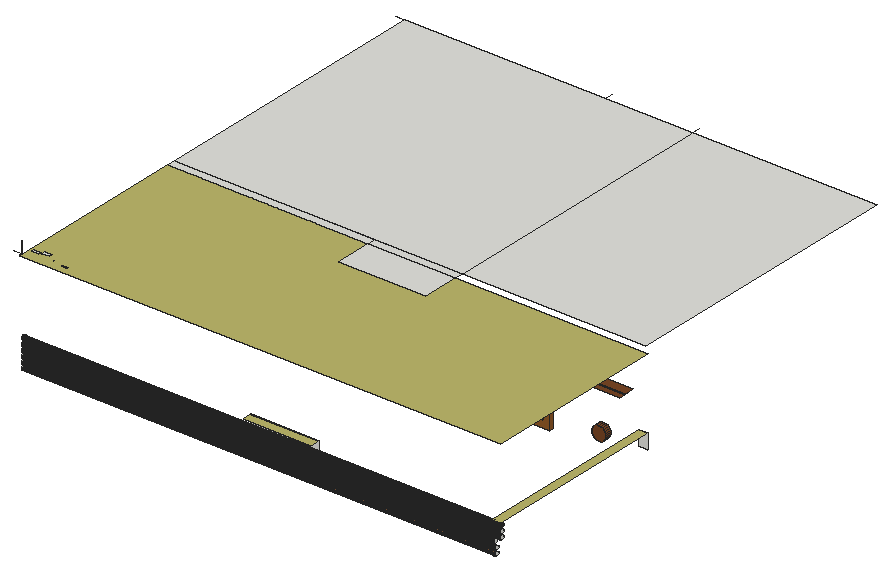
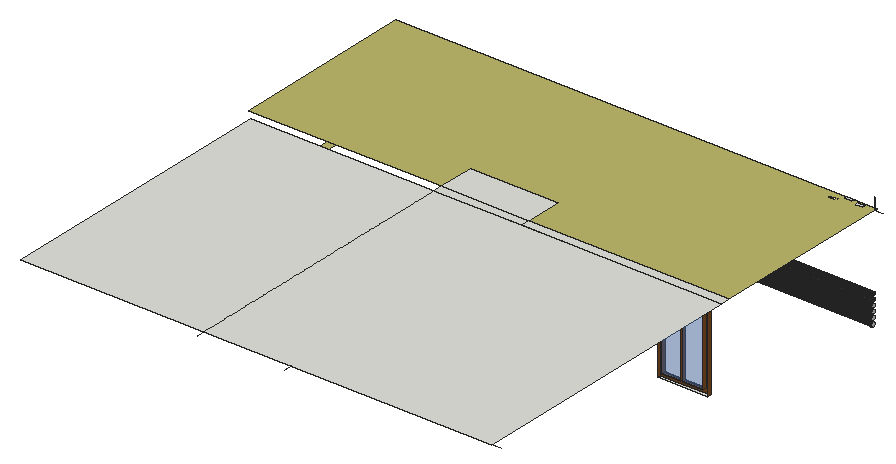
# SketchUp Ruby script. Lengths in inches.
U = 1.inch
M = Sketchup.active_model
def pt(a) = Geom::Point3d.new(a.map { |v| v * U })
def face(e, loops, mat)
  f = e.add_face(loops[0].map { |a| pt(a) })
  loops[1..].each { |l| e.add_face(l.map { |a| pt(a) }).erase! }
  f.material = f.back_material = mat if mat
  f
end
# faces: each face lists its corners as indices into pts; further lists are holes
def faces(e, pts, list, mat = nil) = list.each { |f| face(e, (f[0].is_a?(Array) ? f : [f]).map { |l| l.map { |i| pts[i] } }, mat) }
# xy, xz, yz: faces in a plane at the given z, y or x. An outline is a flat list of corners, or four numbers for a rectangle; further outlines are holes
def ring(l) = l.size == 4 ? [[l[0], l[1]], [l[2], l[1]], [l[2], l[3]], [l[0], l[3]]] : l.each_slice(2).to_a
def flat(e, list, mat, &to3) = list.each { |f| face(e, (f[0].is_a?(Array) ? f : [f]).map { |l| ring(l).map { |u, v| to3.(u, v) } }, mat) }
def xy(e, z, list, mat = nil) = flat(e, list, mat) { |x, y| [x, y, z] }
def xz(e, y, list, mat = nil) = flat(e, list, mat) { |x, z| [x, y, z] }
def yz(e, x, list, mat = nil) = flat(e, list, mat) { |y, z| [x, y, z] }
def lines(e, pts, list) = list.each { |a, b| e.add_line(pt(pts[a]), pt(pts[b])) }
# prism: a flat outline (further loops are holes) pulled along v
def prism(e, loops, v, mat = nil)
  f = face(e, loops, mat); d = Geom::Vector3d.new(v.map { |x| x * U })
  f.pushpull(f.normal.samedirection?(d) ? d.length : -d.length)
end
def box(e, o, s, mat = nil) = prism(e, [[o, [o[0] + s[0], o[1], o[2]], [o[0] + s[0], o[1] + s[1], o[2]], [o[0], o[1] + s[1], o[2]]]], [0, 0, s[2]], mat)
def at(x, y, z, deg = 0) = Geom::Transformation.translation(pt([x, y, z])) * Geom::Transformation.rotation(ORIGIN, Z_AXIS, deg.degrees)
def axes(o, x, y, z) = Geom::Transformation.new([*x, 0, *y, 0, *z, 0, *pt(o).to_a, 1])
def part(name) = M.definitions.add(name)
# library, detail: a bought-in or finely detailed component or shape, given as its bounding box
def library(name, o, s) = part(name).tap { |d| box(d.entities, o, s) }
def detail(e, o, s) = box(e.add_group.entities, o, s)
def put(e, d, t, mat = nil) = e.add_instance(d, t).tap { |i| i.material = mat if mat }
def group(e, t, mat = nil) = e.add_group.tap { |g| g.transformation = t; g.material = mat if mat }.entities
root = M.entities
M.materials.add("[0057_DarkKhaki]").color = [189, 183, 107]
M.materials.add("[Sandstone]").color = [118, 81, 52]
M.materials.add("[Translucent Glass Blue]").color = [100, 149, 237]
M.materials["[Translucent Glass Blue]"].alpha = 0.5
M.materials.add("[Wood Bamboo]").color = [177, 105, 43]
M.materials.add("[Wood Floor Parquet]").color = [145, 89, 39]
M.materials.add("[Wood Veneer 01]").color = [120, 70, 37]
xy(root,380.84,[[312.25,189.3,386.1875,192.3]],"[Wood Floor Parquet]")
xy(root,386.98,[[29.8125,189.3,79,192.3]])
xy(root,387.65,[[319.06,189.3,349.22,192.3],[353.36,189.3,379.38,192.3]],"[Wood Floor Parquet]")
xy(root,391.47,[[34.31,189.3,54.41,192.3],[56.03,189.3,74.5,192.3]],"[Wood Floor Parquet]")
xy(root,396.16,[[109.64,186.3,111.7,189.3]],"[Wood Bamboo]")
xy(root,401.1,[[96.64,186.3,109.64,189.3]],"[Wood Bamboo]")
xy(root,403.6,[[96.64,186.3,111.7,189.3]],"[Wood Bamboo]")
xy(root,410.4375,[[471.0625,12,480,192.3]],"[0057_DarkKhaki]")
xy(root,413.38,[[227.54,12,293.97,21]],"[0057_DarkKhaki]")
xy(root,429.52,[[123.78,186.3,171.53,189.3]],"[Wood Bamboo]")
xy(root,438.4,[[426.75,183.3,426.75,189.3,410.93,189.3,410.93,192.3,459.74,192.3,459.74,189.3,427.96,189.3,427.96,183.3]])
xy(root,438.4,[[410.93,183.3,426.75,189.3],[427.96,183.3,459.74,189.3]],"[Wood Veneer 01]")
xy(root,440.64,[[123.78,186.3,171.53,189.3]],"[Wood Bamboo]")
xy(root,444,[[116.27,186.3,119.49,186.3,119.49,189.3,176.74,189.3,176.74,192.3,92.74,192.3,92.74,189.3,116.27,189.3]],"[Wood Bamboo]")
xy(root,444,[[405.34,183.3,465.34,192.3]],"[Wood Veneer 01]")
xy(root,447.98,[[319.06,189.3,349.22,192.3],[353.36,189.3,379.38,192.3]],"[Wood Floor Parquet]")
xy(root,454.78,[[312.25,189.3,386.1875,192.3]],"[Wood Floor Parquet]")
xy(root,457.11,[[34.31,189.3,54.41,192.3],[56.03,189.3,74.5,192.3]],"[Wood Floor Parquet]")
xy(root,461.6,[[29.8125,189.3,79,192.3]],"[Wood Floor Parquet]")
xy(root,479.9375,[[34.65,18,41.83,21]])
xy(root,480,[[205.37,156.87,290.8125,192.3],[9,192.3,205.37,201.23],[205.37,192.3,290.8125,201.23],[9,201.23,290.8125,483],[290.8125,201.23,471,483]])
xy(root,480,[[[9,12,9,192.3,205.37,192.3,205.37,156.87,290.8125,156.87,290.8125,192.3,480,192.3,480,12],[42.9,18,50.08,21]]],"[0057_DarkKhaki]")
xy(root,483.12,[[15.02,18,22.21,21]])
xy(root,485,[[25.65,18,32.83,21]])
xz(root,21,[[227.54,389.38,293.97,413.38]])
xz(root,183.3,[[438.92,392.76,440.72,393,442.39,393.69,443.83,394.8,444.93,396.23,445.625,397.91,445.86,399.7,445.625,401.5,444.93,403.17,443.83,404.61,442.39,405.71,440.72,406.4,438.92,406.64,437.13,406.4,435.46,405.71,434.02,404.61,432.92,403.17,432.22,401.5,431.99,399.7,432.22,397.91,432.92,396.23,434.02,394.8,435.46,393.69,437.13,393]],"[Wood Veneer 01]")
xz(root,186.3,[[132.85,392.25,134.99,392.53,136.98,393.36,138.68,394.67,140,396.38,140.82,398.37,141.1,400.5,140.82,402.64,140,404.63,138.68,406.34,136.98,407.65,134.99,408.47,132.85,408.75,130.72,408.47,128.73,407.65,127.02,406.34,125.71,404.63,124.88,402.64,124.6,400.5,124.88,398.37,125.71,396.38,127.02,394.67,128.73,393.36,130.72,392.53],[109.64,396.16,111.7,396.16,111.7,403.6,96.64,403.6,96.64,401.1,109.64,401.1],[123.78,429.52,171.53,440.64]],"[Wood Bamboo]")
xz(root,189.3,[[109.64,396.16,109.64,401.1,96.64,401.1,96.64,403.6,111.7,403.6,111.7,396.16]])
xz(root,189.3,[[[119.49,422.86,176.74,444],[123.78,429.52,171.53,440.64]]],"[Wood Bamboo]")
xz(root,189.3,[[[312.25,380.84,386.1875,454.78],[319.06,387.65,349.22,447.98],[353.36,387.65,379.38,447.98]],[[29.8125,386.98,79,461.6],[34.31,391.47,54.41,457.11],[56.03,391.47,74.5,457.11]]],"[Wood Floor Parquet]")
xz(root,192.3,[[[312.25,380.84,386.1875,454.78],[319.06,387.65,349.22,447.98],[353.36,387.65,379.38,447.98]],[471.0625,396,480,410.4375]])
xz(root,192.3,[[319.06,387.65,349.22,447.98],[353.36,387.65,379.38,447.98],[34.31,391.47,54.41,457.11],[56.03,391.47,74.5,457.11]],"[Translucent Glass Blue]")
yz(root,9,[[15.36,378.27,14.91,378.33,14.49,378.5,14.125,378.78,13.85,379.14,13.67,379.5625,13.61,380.02,13.67,380.47,13.85,380.89,14.125,381.25,14.49,381.53,14.91,381.71,15.36,381.77,15.82,381.71,16.24,381.53,16.6,381.25,16.88,380.89,17.05,380.47,17.11,380.02,17.05,379.5625,16.88,379.14,16.6,378.78,16.24,378.5,15.82,378.33],[15.36,383.58,14.91,383.64,14.49,383.8125,14.125,384.09,13.85,384.45,13.67,384.875,13.61,385.33,13.67,385.78,13.85,386.2,14.125,386.57,14.49,386.84,14.91,387.02,15.36,387.08,15.82,387.02,16.24,386.84,16.6,386.57,16.88,386.2,17.05,385.78,17.11,385.33,17.05,384.875,16.88,384.45,16.6,384.09,16.24,383.8125,15.82,383.64],[15.36,388.89,14.91,388.95,14.49,389.125,14.125,389.4,13.85,389.77,13.67,390.1875,13.61,390.64,13.67,391.09,13.85,391.52,14.125,391.88,14.49,392.16,14.91,392.33,15.36,392.39,15.82,392.33,16.24,392.16,16.6,391.88,16.88,391.52,17.05,391.09,17.11,390.64,17.05,390.1875,16.88,389.77,16.6,389.4,16.24,389.125,15.82,388.95],[15.36,394.2,14.91,394.26,14.49,394.4375,14.125,394.72,13.85,395.08,13.67,395.5,13.61,395.95,13.67,396.41,13.85,396.83,14.125,397.19,14.49,397.47,14.91,397.64,15.36,397.7,15.82,397.64,16.24,397.47,16.6,397.19,16.88,396.83,17.05,396.41,17.11,395.95,17.05,395.5,16.88,395.08,16.6,394.72,16.24,394.4375,15.82,394.26]])
yz(root,29.8125,[[189.3,386.98,192.3,461.6]],"[Wood Floor Parquet]")
yz(root,34.31,[[189.3,391.47,192.3,457.11]],"[Wood Floor Parquet]")
yz(root,54.41,[[189.3,391.47,192.3,457.11]],"[Wood Floor Parquet]")
yz(root,56.03,[[189.3,391.47,192.3,457.11]],"[Wood Floor Parquet]")
yz(root,74.5,[[189.3,391.47,192.3,457.11]],"[Wood Floor Parquet]")
yz(root,79,[[189.3,386.98,192.3,461.6]],"[Wood Floor Parquet]")
yz(root,96.64,[[186.3,401.1,189.3,403.6]],"[Wood Bamboo]")
yz(root,109.64,[[186.3,396.16,189.3,401.1]],"[Wood Bamboo]")
yz(root,111.7,[[186.3,396.16,189.3,403.6]],"[Wood Bamboo]")
yz(root,123.78,[[186.3,429.52,189.3,440.64]],"[Wood Bamboo]")
yz(root,171.53,[[186.3,429.52,189.3,440.64]],"[Wood Bamboo]")
yz(root,312.25,[[189.3,380.84,192.3,454.78]],"[Wood Floor Parquet]")
yz(root,319.06,[[189.3,387.65,192.3,447.98]],"[Wood Floor Parquet]")
yz(root,349.22,[[189.3,387.65,192.3,447.98]],"[Wood Floor Parquet]")
yz(root,353.36,[[189.3,387.65,192.3,447.98]],"[Wood Floor Parquet]")
yz(root,379.38,[[189.3,387.65,192.3,447.98]],"[Wood Floor Parquet]")
yz(root,386.1875,[[189.3,380.84,192.3,454.78]],"[Wood Floor Parquet]")
yz(root,472.25,[[15.36,388.89,15.82,388.95,16.24,389.125,16.6,389.4,16.88,389.77,17.05,390.1875,17.11,390.64,17.05,391.09,16.88,391.52,16.6,391.88,16.24,392.16,15.82,392.33,15.36,392.39,14.91,392.33,14.49,392.16,14.125,391.88,13.85,391.52,13.67,391.09,13.61,390.64,13.67,390.1875,13.85,389.77,14.125,389.4,14.49,389.125,14.91,388.95]])
yz(root,473.625,[[15.36,378.27,15.82,378.33,16.24,378.5,16.6,378.78,16.88,379.14,17.05,379.5625,17.11,380.02,17.05,380.47,16.88,380.89,16.6,381.25,16.24,381.53,15.82,381.71,15.36,381.77,14.91,381.71,14.49,381.53,14.125,381.25,13.85,380.89,13.67,380.47,13.61,380.02,13.67,379.5625,13.85,379.14,14.125,378.78,14.49,378.5,14.91,378.33],[15.36,383.58,15.82,383.64,16.24,383.8125,16.6,384.09,16.88,384.45,17.05,384.875,17.11,385.33,17.05,385.78,16.88,386.2,16.6,386.57,16.24,386.84,15.82,387.02,15.36,387.08,14.91,387.02,14.49,386.84,14.125,386.57,13.85,386.2,13.67,385.78,13.61,385.33,13.67,384.875,13.85,384.45,14.125,384.09,14.49,383.8125,14.91,383.64]])
yz(root,478.4375,[[15.36,394.2,15.82,394.26,16.24,394.4375,16.6,394.72,16.88,395.08,17.05,395.5,17.11,395.95,17.05,396.41,16.88,396.83,16.6,397.19,16.24,397.47,15.82,397.64,15.36,397.7,14.91,397.64,14.49,397.47,14.125,397.19,13.85,396.83,13.67,396.41,13.61,395.95,13.67,395.5,13.85,395.08,14.125,394.72,14.49,394.4375,14.91,394.26],[15.36,399.52,15.82,399.58,16.24,399.75,16.6,400.03,16.88,400.39,17.05,400.8125,17.11,401.27,17.05,401.72,16.88,402.14,16.6,402.5,16.24,402.78,15.82,402.96,15.36,403.02,14.91,402.96,14.49,402.78,14.125,402.5,13.85,402.14,13.67,401.72,13.61,401.27,13.67,400.8125,13.85,400.39,14.125,400.03,14.49,399.75,14.91,399.58]])
p = [[9,14.49,378.5],[9,14.91,378.33],[473.625,14.91,378.33],[473.625,14.49,378.5],[9,15.36,378.27],[473.625,15.36,378.27],
  [9,15.82,378.33],[473.625,15.82,378.33],[9,16.24,378.5],[473.625,16.24,378.5],[9,14.125,378.78],[473.625,14.125,378.78],
  [9,16.6,378.78],[473.625,16.6,378.78],[9,13.85,379.14],[473.625,13.85,379.14],[9,16.88,379.14],[473.625,16.88,379.14],
  [9,13.67,379.5625],[473.625,13.67,379.5625],[9,17.05,379.5625],[473.625,17.05,379.5625],[9,13.61,380.02],[473.625,13.61,380.02],
  [9,17.11,380.02],[473.625,17.11,380.02],[9,13.67,380.47],[473.625,13.67,380.47],[9,17.05,380.47],[473.625,17.05,380.47],
  [9,13.85,380.89],[473.625,13.85,380.89],[9,16.88,380.89],[473.625,16.88,380.89],[9,14.125,381.25],[473.625,14.125,381.25],
  [9,16.6,381.25],[473.625,16.6,381.25],[9,14.49,381.53],[473.625,14.49,381.53],[9,16.24,381.53],[473.625,16.24,381.53],
  [9,14.91,381.71],[473.625,14.91,381.71],[9,15.82,381.71],[473.625,15.82,381.71],[9,15.36,381.77],[473.625,15.36,381.77],
  [9,14.49,383.8125],[9,14.91,383.64],[473.625,14.91,383.64],[473.625,14.49,383.8125],[9,15.36,383.58],[473.625,15.36,383.58],
  [9,15.82,383.64],[473.625,15.82,383.64],[9,16.24,383.8125],[473.625,16.24,383.8125],[9,14.125,384.09],[473.625,14.125,384.09],
  [9,16.6,384.09],[473.625,16.6,384.09],[9,13.85,384.45],[473.625,13.85,384.45],[9,16.88,384.45],[473.625,16.88,384.45],
  [9,13.67,384.875],[473.625,13.67,384.875],[9,17.05,384.875],[473.625,17.05,384.875],[9,13.61,385.33],[473.625,13.61,385.33],
  [9,17.11,385.33],[473.625,17.11,385.33],[9,13.67,385.78],[473.625,13.67,385.78],[9,17.05,385.78],[473.625,17.05,385.78],
  [9,13.85,386.2],[473.625,13.85,386.2],[9,16.88,386.2],[473.625,16.88,386.2],[9,14.125,386.57],[473.625,14.125,386.57],
  [9,16.6,386.57],[473.625,16.6,386.57],[9,14.49,386.84],[473.625,14.49,386.84],[9,16.24,386.84],[473.625,16.24,386.84],
  [9,14.91,387.02],[473.625,14.91,387.02],[9,15.82,387.02],[473.625,15.82,387.02],[9,15.36,387.08],[473.625,15.36,387.08],
  [9,14.91,388.95],[9,15.36,388.89],[472.25,15.36,388.89],[472.25,14.91,388.95],[9,15.82,388.95],[472.25,15.82,388.95],
  [9,14.49,389.125],[472.25,14.49,389.125],[9,16.24,389.125],[472.25,16.24,389.125],[9,14.125,389.4],[472.25,14.125,389.4],
  [9,16.6,389.4],[472.25,16.6,389.4],[9,13.85,389.77],[472.25,13.85,389.77],[9,16.88,389.77],[472.25,16.88,389.77],
  [9,13.67,390.1875],[472.25,13.67,390.1875],[9,17.05,390.1875],[472.25,17.05,390.1875],[9,13.61,390.64],[472.25,13.61,390.64],
  [9,17.11,390.64],[472.25,17.11,390.64],[9,13.67,391.09],[472.25,13.67,391.09],[9,17.05,391.09],[472.25,17.05,391.09],
  [9,13.85,391.52],[472.25,13.85,391.52],[9,16.88,391.52],[472.25,16.88,391.52],[9,14.125,391.88],[472.25,14.125,391.88],
  [9,16.6,391.88],[472.25,16.6,391.88],[9,14.49,392.16],[472.25,14.49,392.16],[9,16.24,392.16],[472.25,16.24,392.16],
  [9,14.91,392.33],[472.25,14.91,392.33],[9,15.82,392.33],[472.25,15.82,392.33],[9,15.36,392.39],[472.25,15.36,392.39],
  [130.72,189.3,392.53],[132.85,189.3,392.25],[132.85,186.3,392.25],[130.72,186.3,392.53],[134.99,189.3,392.53],[134.99,186.3,392.53],
  [128.73,189.3,393.36],[128.73,186.3,393.36],[136.98,189.3,393.36],[136.98,186.3,393.36],[437.13,189.3,393],[438.92,189.3,392.76],
  [438.92,183.3,392.76],[437.13,183.3,393],[440.72,189.3,393],[440.72,183.3,393],[435.46,189.3,393.69],[435.46,183.3,393.69],
  [442.39,189.3,393.69],[442.39,183.3,393.69],[127.02,189.3,394.67],[127.02,186.3,394.67],[138.68,189.3,394.67],[138.68,186.3,394.67],
  [434.02,189.3,394.8],[434.02,183.3,394.8],[443.83,189.3,394.8],[443.83,183.3,394.8],[9,14.91,394.26],[9,15.36,394.2],
  [478.4375,15.36,394.2],[478.4375,14.91,394.26],[9,15.82,394.26],[478.4375,15.82,394.26],[9,14.49,394.4375],[478.4375,14.49,394.4375],
  [9,16.24,394.4375],[478.4375,16.24,394.4375],[9,14.125,394.72],[478.4375,14.125,394.72],[9,16.6,394.72],[478.4375,16.6,394.72],
  [9,13.85,395.08],[478.4375,13.85,395.08],[9,16.88,395.08],[478.4375,16.88,395.08],[125.71,189.3,396.38],[125.71,186.3,396.38],
  [140,189.3,396.38],[140,186.3,396.38],[432.92,189.3,396.23],[432.92,183.3,396.23],[444.93,189.3,396.23],[444.93,183.3,396.23],
  [9,13.67,395.5],[478.4375,13.67,395.5],[9,17.05,395.5],[478.4375,17.05,395.5],[9,13.61,395.95],[478.4375,13.61,395.95],
  [9,17.11,395.95],[478.4375,17.11,395.95],[9,13.67,396.41],[478.4375,13.67,396.41],[9,17.05,396.41],[478.4375,17.05,396.41],
  [432.22,189.3,397.91],[432.22,183.3,397.91],[445.625,189.3,397.91],[445.625,183.3,397.91],[9,13.85,396.83],[478.4375,13.85,396.83],
  [9,16.88,396.83],[478.4375,16.88,396.83],[124.88,189.3,398.37],[124.88,186.3,398.37],[140.82,189.3,398.37],[140.82,186.3,398.37],
  [9,14.125,397.19],[478.4375,14.125,397.19],[9,16.6,397.19],[478.4375,16.6,397.19],[9,14.49,397.47],[478.4375,14.49,397.47],
  [9,16.24,397.47],[478.4375,16.24,397.47],[9,14.91,397.64],[478.4375,14.91,397.64],[9,15.82,397.64],[478.4375,15.82,397.64],
  [9,15.36,397.7],[478.4375,15.36,397.7],[431.99,189.3,399.7],[431.99,183.3,399.7],[445.86,189.3,399.7],[445.86,183.3,399.7],
  [124.6,189.3,400.5],[124.6,186.3,400.5],[141.1,189.3,400.5],[141.1,186.3,400.5],[9,14.91,399.58],[9,15.36,399.52],
  [478.4375,15.36,399.52],[478.4375,14.91,399.58],[9,15.82,399.58],[478.4375,15.82,399.58],[9,14.49,399.75],[478.4375,14.49,399.75],
  [9,16.24,399.75],[478.4375,16.24,399.75],[432.22,189.3,401.5],[432.22,183.3,401.5],[445.625,189.3,401.5],[445.625,183.3,401.5],
  [9,14.125,400.03],[478.4375,14.125,400.03],[9,16.6,400.03],[478.4375,16.6,400.03],[9,13.85,400.39],[478.4375,13.85,400.39],
  [9,16.88,400.39],[478.4375,16.88,400.39],[9,13.67,400.8125],[478.4375,13.67,400.8125],[9,17.05,400.8125],[478.4375,17.05,400.8125],
  [124.88,189.3,402.64],[124.88,186.3,402.64],[140.82,189.3,402.64],[140.82,186.3,402.64],[9,13.61,401.27],[478.4375,13.61,401.27],
  [9,17.11,401.27],[478.4375,17.11,401.27],[9,13.67,401.72],[478.4375,13.67,401.72],[9,17.05,401.72],[478.4375,17.05,401.72],
  [432.92,189.3,403.17],[432.92,183.3,403.17],[444.93,189.3,403.17],[444.93,183.3,403.17],[9,13.85,402.14],[478.4375,13.85,402.14],
  [9,16.88,402.14],[478.4375,16.88,402.14],[9,14.125,402.5],[478.4375,14.125,402.5],[9,16.6,402.5],[478.4375,16.6,402.5],
  [9,14.49,402.78],[478.4375,14.49,402.78],[9,16.24,402.78],[478.4375,16.24,402.78],[125.71,189.3,404.63],[125.71,186.3,404.63],
  [140,189.3,404.63],[140,186.3,404.63],[9,14.91,402.96],[478.4375,14.91,402.96],[9,15.82,402.96],[478.4375,15.82,402.96],
  [9,15.36,403.02],[478.4375,15.36,403.02],[434.02,189.3,404.61],[434.02,183.3,404.61],[443.83,189.3,404.61],[443.83,183.3,404.61],
  [435.46,189.3,405.71],[435.46,183.3,405.71],[442.39,189.3,405.71],[442.39,183.3,405.71],[127.02,189.3,406.34],[127.02,186.3,406.34],
  [138.68,189.3,406.34],[138.68,186.3,406.34],[9,14.49,405.1875],[9,14.91,405.01],[478.4375,14.91,405.01],[478.4375,14.49,405.1875],
  [9,15.36,404.95],[478.4375,15.36,404.95],[9,15.82,405.01],[478.4375,15.82,405.01],[9,16.24,405.1875],[478.4375,16.24,405.1875],
  [9,14.125,405.47],[478.4375,14.125,405.47],[9,16.6,405.47],[478.4375,16.6,405.47],[9,13.85,405.83],[478.4375,13.85,405.83],
  [9,16.88,405.83],[478.4375,16.88,405.83],[437.13,189.3,406.4],[437.13,183.3,406.4],[440.72,189.3,406.4],[440.72,183.3,406.4],
  [9,13.67,406.25],[478.4375,13.67,406.25],[9,17.05,406.25],[478.4375,17.05,406.25],[9,13.61,406.7],[478.4375,13.61,406.7],
  [9,17.11,406.7],[478.4375,17.11,406.7],[128.73,189.3,407.65],[128.73,186.3,407.65],[136.98,189.3,407.65],[136.98,186.3,407.65],
  [438.92,189.3,406.64],[438.92,183.3,406.64],[9,13.67,407.16],[478.4375,13.67,407.16],[9,17.05,407.16],[478.4375,17.05,407.16],
  [9,13.85,407.58],[478.4375,13.85,407.58],[9,16.88,407.58],[478.4375,16.88,407.58],[9,14.125,407.94],[478.4375,14.125,407.94],
  [9,16.6,407.94],[478.4375,16.6,407.94],[130.72,189.3,408.47],[130.72,186.3,408.47],[134.99,189.3,408.47],[134.99,186.3,408.47],
  [9,14.49,408.22],[478.4375,14.49,408.22],[9,16.24,408.22],[478.4375,16.24,408.22],[9,14.91,408.39],[478.4375,14.91,408.39],
  [9,15.82,408.39],[478.4375,15.82,408.39],[9,15.36,408.45],[478.4375,15.36,408.45],[132.85,189.3,408.75],[132.85,186.3,408.75],
  [9,14.8125,480],[9,14.8125,492],[205.37,483,480],[205.37,492,480],[9,483,480],[0,483,480],
  [7.75,14.8125,480],[290.8125,483,480],[290.8125,492,480],[7.75,12,480],[7.75,14.8125,492],[0,14.8125,480]]
faces(root,p,[[0,1,2,3],[1,4,5,2],[4,6,7,5],[6,8,9,7],[10,0,3,11],[8,12,13,9],[14,10,11,15],[12,16,17,13],
  [18,14,15,19],[16,20,21,17],[22,18,19,23],[20,24,25,21],[26,22,23,27],[24,28,29,25],[30,26,27,31],[28,32,33,29],
  [34,30,31,35],[32,36,37,33],[38,34,35,39],[36,40,41,37],[42,38,39,43],[40,44,45,41],[46,42,43,47],[44,46,47,45],
  [48,49,50,51],[49,52,53,50],[52,54,55,53],[54,56,57,55],[58,48,51,59],[56,60,61,57],[62,58,59,63],[60,64,65,61],
  [66,62,63,67],[64,68,69,65],[70,66,67,71],[68,72,73,69],[74,70,71,75],[72,76,77,73],[78,74,75,79],[76,80,81,77],
  [82,78,79,83],[80,84,85,81],[86,82,83,87],[84,88,89,85],[90,86,87,91],[88,92,93,89],[94,90,91,95],[92,94,95,93],
  [96,97,98,99],[97,100,101,98],[102,96,99,103],[100,104,105,101],[106,102,103,107],[104,108,109,105],[110,106,107,111],[108,112,113,109],
  [114,110,111,115],[112,116,117,113],[118,114,115,119],[116,120,121,117],[122,118,119,123],[120,124,125,121],[126,122,123,127],[124,128,129,125],
  [130,126,127,131],[128,132,133,129],[134,130,131,135],[132,136,137,133],[138,134,135,139],[136,140,141,137],[142,138,139,143],[140,142,143,141],
  [172,173,174,175],[173,176,177,174],[178,172,175,179],[176,180,181,177],[182,178,179,183],[180,184,185,181],[186,182,183,187],[184,188,189,185],
  [198,186,187,199],[188,200,201,189],[202,198,199,203],[200,204,205,201],[206,202,203,207],[204,208,209,205],[214,206,207,215],[208,216,217,209],
  [222,214,215,223],[216,224,225,217],[226,222,223,227],[224,228,229,225],[230,226,227,231],[228,232,233,229],[234,230,231,235],[232,234,235,233],
  [244,245,246,247],[245,248,249,246],[250,244,247,251],[248,252,253,249],[258,250,251,259],[252,260,261,253],[262,258,259,263],[260,264,265,261],
  [266,262,263,267],[264,268,269,265],[274,266,267,275],[268,276,277,269],[278,274,275,279],[276,280,281,277],[286,278,279,287],[280,288,289,281],
  [290,286,287,291],[288,292,293,289],[294,290,291,295],[292,296,297,293],[302,294,295,303],[296,304,305,297],[306,302,303,307],[304,306,307,305],
  [320,321,322,323],[321,324,325,322],[324,326,327,325],[326,328,329,327],[330,320,323,331],[328,332,333,329],[334,330,331,335],[332,336,337,333],
  [342,334,335,343],[336,344,345,337],[346,342,343,347],[344,348,349,345],[356,346,347,357],[348,358,359,349],[360,356,357,361],[358,362,363,359],
  [364,360,361,365],[362,366,367,363],[372,364,365,373],[366,374,375,367],[376,372,373,377],[374,378,379,375],[380,376,377,381],[378,380,381,379]],"[Sandstone]")
faces(root,p,[[144,145,146,147],[145,148,149,146],[150,144,147,151],[148,152,153,149],[164,150,151,165],[152,166,167,153],[190,164,165,191],[166,192,193,167],
  [218,190,191,219],[192,220,221,193],[240,218,219,241],[220,242,243,221],[270,240,241,271],[242,272,273,243],[298,270,271,299],[272,300,301,273],
  [316,298,299,317],[300,318,319,301],[350,316,317,351],[318,352,353,319],[368,350,351,369],[352,370,371,353],[382,368,369,383],[370,382,383,371]],"[Wood Bamboo]")
faces(root,p,[[154,155,156,157],[155,158,159,156],[160,154,157,161],[158,162,163,159],[168,160,161,169],[162,170,171,163],[194,168,169,195],[170,196,197,171],
  [210,194,195,211],[196,212,213,197],[236,210,211,237],[212,238,239,213],[254,236,237,255],[238,256,257,239],[282,254,255,283],[256,284,285,257],
  [308,282,283,309],[284,310,311,285],[312,308,309,313],[310,314,315,311],[338,312,313,339],[314,340,341,315],[354,338,339,355],[340,354,355,341]],"[Wood Veneer 01]")
lines(root,p,[[384,385],[386,387],[388,389],[384,390],[391,392],[390,393],[390,394],[390,395]])
